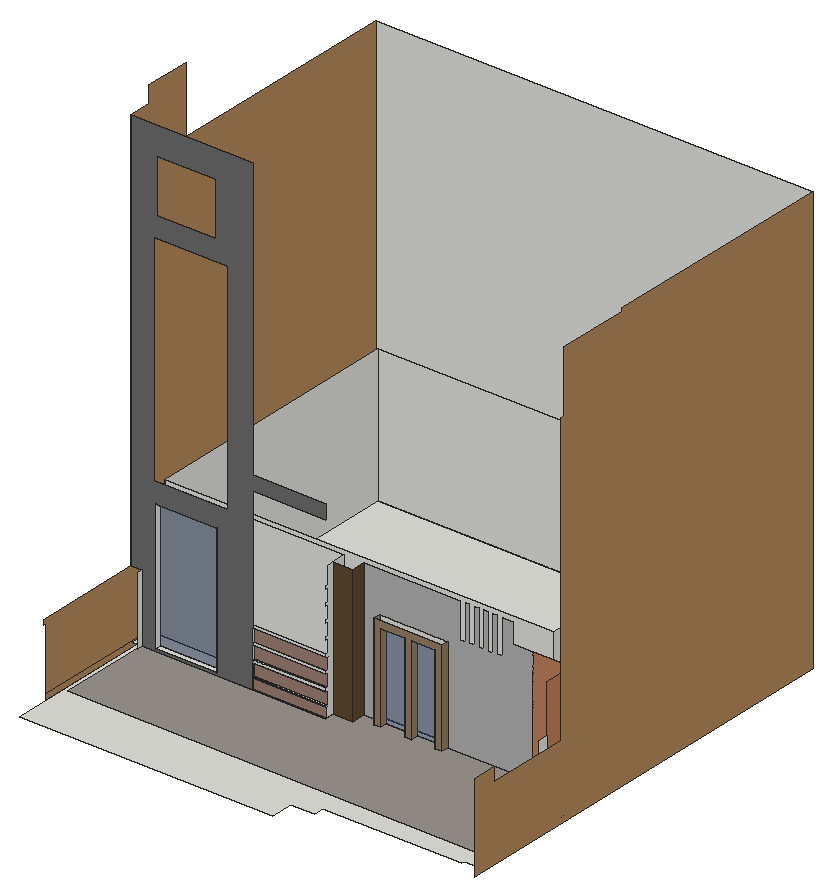
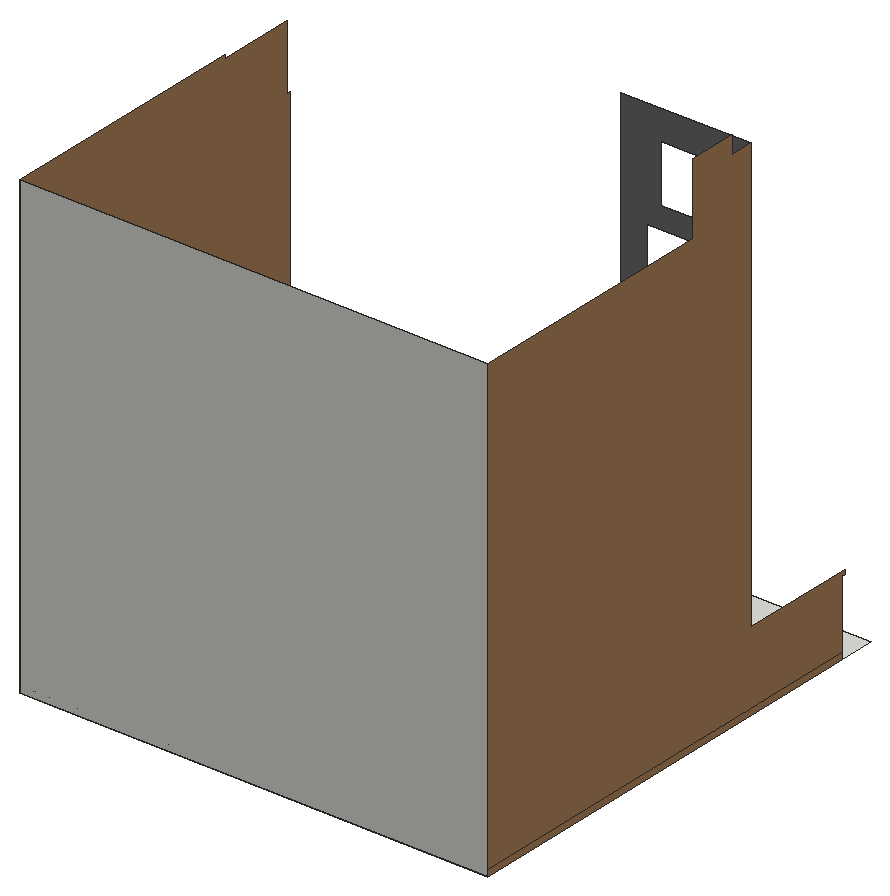
# SketchUp Ruby script. Lengths in inches.
U = 1.inch
M = Sketchup.active_model
def pt(a) = Geom::Point3d.new(a.map { |v| v * U })
def face(e, loops, mat)
  f = e.add_face(loops[0].map { |a| pt(a) })
  loops[1..].each { |l| e.add_face(l.map { |a| pt(a) }).erase! }
  f.material = f.back_material = mat if mat
  f
end
# faces: each face lists its corners as indices into pts; further lists are holes
def faces(e, pts, list, mat = nil) = list.each { |f| face(e, (f[0].is_a?(Array) ? f : [f]).map { |l| l.map { |i| pts[i] } }, mat) }
# xy, xz, yz: faces in a plane at the given z, y or x. An outline is a flat list of corners, or four numbers for a rectangle; further outlines are holes
def ring(l) = l.size == 4 ? [[l[0], l[1]], [l[2], l[1]], [l[2], l[3]], [l[0], l[3]]] : l.each_slice(2).to_a
def flat(e, list, mat, &to3) = list.each { |f| face(e, (f[0].is_a?(Array) ? f : [f]).map { |l| ring(l).map { |u, v| to3.(u, v) } }, mat) }
def xy(e, z, list, mat = nil) = flat(e, list, mat) { |x, y| [x, y, z] }
def xz(e, y, list, mat = nil) = flat(e, list, mat) { |x, z| [x, y, z] }
def yz(e, x, list, mat = nil) = flat(e, list, mat) { |y, z| [x, y, z] }
def lines(e, pts, list) = list.each { |a, b| e.add_line(pt(pts[a]), pt(pts[b])) }
# prism: a flat outline (further loops are holes) pulled along v
def prism(e, loops, v, mat = nil)
  f = face(e, loops, mat); d = Geom::Vector3d.new(v.map { |x| x * U })
  f.pushpull(f.normal.samedirection?(d) ? d.length : -d.length)
end
def box(e, o, s, mat = nil) = prism(e, [[o, [o[0] + s[0], o[1], o[2]], [o[0] + s[0], o[1] + s[1], o[2]], [o[0], o[1] + s[1], o[2]]]], [0, 0, s[2]], mat)
def at(x, y, z, deg = 0) = Geom::Transformation.translation(pt([x, y, z])) * Geom::Transformation.rotation(ORIGIN, Z_AXIS, deg.degrees)
def axes(o, x, y, z) = Geom::Transformation.new([*x, 0, *y, 0, *z, 0, *pt(o).to_a, 1])
def part(name) = M.definitions.add(name)
# library, detail: a bought-in or finely detailed component or shape, given as its bounding box
def library(name, o, s) = part(name).tap { |d| box(d.entities, o, s) }
def detail(e, o, s) = box(e.add_group.entities, o, s)
def put(e, d, t, mat = nil) = e.add_instance(d, t).tap { |i| i.material = mat if mat }
def group(e, t, mat = nil) = e.add_group.tap { |g| g.transformation = t; g.material = mat if mat }.entities
root = M.entities
M.materials.add("Niraj_Hair_Dark").color = [109, 109, 109]
M.materials.add("Niraj_Hair_Gray").color = [178, 178, 178]
M.materials.add("Niraj_Shoe_Sole").color = [96, 73, 48]
M.materials.add("Niraj_Shoe_Stitching").color = [181, 137, 92]
M.materials.add("Niraj_Skin").color = [158, 128, 115]
M.materials.add("[0035_Tan]").color = [150, 128, 100]
M.materials.add("[Granite Tile]").color = [155, 148, 143]
M.materials.add("[Translucent Glass Blue]").color = [40, 60, 96]
M.materials["[Translucent Glass Blue]"].alpha = 0.5
M.materials.add("[Translucent Glass Blue]1").color = [46, 68, 109]
M.materials["[Translucent Glass Blue]1"].alpha = 0.5
M.materials.add("[Wood Veneer 02]").color = [190, 128, 91]
xy(root,-4.9375,[[0,0,0,391.875,372,391.875,372,115,384,115,384,31.875,365.58,31.875,365.58,28.875,243.65,28.875,243.65,19.875,222.65,19.875,222.65,0],[372,115,384,118],[372,118,384,142],[372,142,372,143.6875,373.25,143.6875,373.25,391.875,384,391.875,384,142],[372,143.6875,373.25,391.875]])
xy(root,0,[[0,122.375,9,142],[9,122.375,106.63,122.375,106.63,123.4375,171.63,123.4375,171.63,142,9,142],[106.63,122.375,171.63,123.1875],[106.63,123.1875,171.63,123.4375],[202.6,136,203.04,142],
  [203.04,136,208.6,142],[229.96,136,231.09,142],[231.09,136,235.96,142],[256.6,136,262.6,142],[262.6,142,337.38,143.6875],
  [337.38,142,360,143.6875],[360,142,360.25,143.6875],[360.25,142,372,143.6875],[262.6,143.6875,337.38,148],[9,148,262.6,382.875],
  [262.6,148,337.38,382.875],[337.38,148,351,382.875]])
xy(root,0,[[9,40.875,375,40.875,375,106,372,106,372,142,262.6,142,262.6,136,256.6,136,256.6,142,235.96,142,235.96,136,229.96,136,229.96,142,208.6,142,208.6,136,202.6,136,202.6,142,189.04,142,189.04,130,171.63,130,171.63,122.375,9,122.375]],"[Granite Tile]")
xy(root,2,[[21.24,122.375,75.18,127.1875]])
xy(root,9.02,[[106.63,122.375,171.63,123.1875]])
xy(root,10.2,[[106.63,122.375,171.63,123.625],[106.63,123.625,171.63,123.75]])
xy(root,21.27,[[106.63,122.375,171.63,123.625],[106.63,123.625,171.63,123.75]])
xy(root,23.7,[[106.63,122.375,171.63,124.125],[106.63,124.125,171.63,124.1875]])
xy(root,34.77,[[106.63,122.375,171.63,124.125],[106.63,124.125,171.63,124.1875]])
xy(root,37.2,[[106.63,122.375,171.63,123.5625]])
xy(root,48.27,[[106.63,122.375,171.63,123.5625]])
xz(root,122.375,[[106.63,-2.05,171.63,0],[106.63,9.02,171.63,10.2],[106.63,21.27,171.63,23.7],[106.63,34.77,171.63,37.2],[106.63,48.27,171.63,50.7]])
xz(root,122.375,[[[9,0,106.63,0,106.63,156.27,171.63,156.27,171.63,169.15,106.63,169.15,106.63,415.46,0,415.46,0,60,9,60],[20.16,134.02,85.33,326.3125],[21.24,2,75.18,116.62],[22.76,343.6,74.01,391.1]]],"Niraj_Hair_Dark")
xz(root,123.1875,[[106.63,0,171.63,9.02]],"Niraj_Skin")
xz(root,123.5625,[[106.63,37.2,171.63,48.27]],"Niraj_Skin")
xz(root,123.75,[[106.63,10.2,171.63,21.27]],"Niraj_Skin")
xz(root,124.1875,[[106.63,23.7,171.63,34.77]],"Niraj_Skin")
xz(root,127.1875,[[21.24,2,75.18,116.62]],"[Translucent Glass Blue]")
xz(root,130,[[171.63,0,189.04,120]],"Niraj_Shoe_Sole")
xz(root,136,[[202.6,0,208.6,0,208.6,78,229.96,78,229.96,0,235.96,0,235.96,78,256.6,78,256.6,0,262.6,0,262.6,84,202.6,84]],"[0035_Tan]")
xz(root,142,[[9,0,171.63,120],[202.6,0,202.6,84,262.6,84,262.6,0,256.6,0,256.6,78,235.96,78,235.96,0,229.96,0,229.96,78,208.6,78,208.6,0]])
xz(root,142,[[189.04,0,202.6,0,202.6,84,262.6,84,262.6,0,337.38,0,337.38,102.25,320.38,102.25,320.38,120,311.1,120,311.1,89.375,306.22,89.375,306.22,120,302.91,120,302.91,89.375,298.04,89.375,298.04,120,294.72,120,294.72,89.375,289.85,89.375,289.85,120,286.54,120,286.54,89.375,281.66,89.375,281.66,120,278.35,120,278.35,89.375,273.47,89.375,273.47,120,189.04,120]],"Niraj_Hair_Gray")
xz(root,142,[[208.6,0,229.96,78],[235.96,0,256.6,78]],"[Translucent Glass Blue]1")
xz(root,142,[[337.38,0,372,102.25]],"[Wood Veneer 02]")
xz(root,143.6875,[[372,-4.9375,373.25,0]])
xz(root,148,[[9,0,351,120]])
xz(root,382.875,[[9,-4.9375,262.6,0],[9,0,351,120]])
xz(root,391.875,[[0,-4.9375,384,371.75]])
yz(root,0,[[28.875,-4.9375,391.875,0],[28.875,0,28.875,56.2,25.875,56.2,25.875,60,122.375,60,122.375,415.46,142,415.46,142,430.21,182.0625,430.21,182.0625,371.75,391.875,371.75,391.875,0]],"Niraj_Shoe_Stitching")
yz(root,9,[[117.875,0,122.375,60],[148,0,382.875,120]])
yz(root,21.24,[[122.375,2,127.1875,116.62]])
yz(root,75.18,[[122.375,2,127.1875,116.62]])
yz(root,106.63,[[122.375,0,123.1875,9.02],[123.1875,0,123.4375,9.02],[122.375,10.2,123.625,21.27],[123.625,10.2,123.75,21.27],[122.375,23.7,124.125,34.77],
  [124.125,23.7,124.1875,34.77],[122.375,37.2,123.5625,48.27],[123.5625,37.2,124.25,48.27]])
yz(root,171.63,[[123.1875,0,130,0,130,120,123.6875,120,123.6875,118.2,124.1875,118.2,124.1875,104.7,122.375,104.7,122.375,102.27,123.5,102.27,123.5,91.2,122.375,91.2,122.375,88.77,123.5625,88.77,123.5625,77.7,122.375,77.7,122.375,75.27,123.875,75.27,123.875,64.2,122.375,64.2,122.375,61.77,124.5,61.77,124.5,50.7,122.375,50.7,122.375,48.27,123.5625,48.27,123.5625,37.2,122.375,37.2,122.375,34.77,124.1875,34.77,124.1875,23.7,122.375,23.7,122.375,21.27,123.75,21.27,123.75,10.2,122.375,10.2,122.375,9.02,123.1875,9.02],[130,0,142,120]])
yz(root,189.04,[[130,0,142,120]],"Niraj_Shoe_Sole")
yz(root,202.6,[[136,0,142,84]],"[0035_Tan]")
yz(root,208.6,[[136,0,142,78]],"[0035_Tan]")
yz(root,229.96,[[136,0,142,78]],"[0035_Tan]")
yz(root,235.96,[[136,0,142,78]],"[0035_Tan]")
yz(root,256.6,[[136,0,142,78]],"[0035_Tan]")
yz(root,262.6,[[136,0,142,84]],"[0035_Tan]")
yz(root,351,[[148,0,382.875,120]])
yz(root,372,[[115,-4.9375,118,0],[118,-4.9375,142,0],[142,-4.9375,143.6875,0],[106,0,115,60],[142,0,143.6875,0.625]])
yz(root,372,[[115,0,142,102.25]],"[Wood Veneer 02]")
yz(root,384,[[19.875,-4.9375,391.875,-4.9375,391.875,371.75,182.0625,371.75,182.0625,369.0625,118,369.0625,118,314.9,115,314.9,115,60,40.875,60,40.875,72,19.875,72]],"Niraj_Shoe_Stitching")
p = [[106.63,124.25,48.27],[171.63,124.25,48.27],[106.63,123.4375,9.02],[171.63,123.4375,9.02],[372,118,0],[384,118,0],
  [360,143.6875,0],[360,391.875,0],[337.38,382.875,0],[337.38,391.875,0],[262.6,382.875,0],[262.6,391.875,0],
  [372,143.6875,0.625],[372,391.875,0.625],[373.25,143.6875,0],[373.25,391.875,0],[9,148,0],[9,148,-4.9375],
  [9,117.875,0],[9,117.875,-4.9375],[9,142,0],[9,142,-4.9375],[262.6,382.875,-4.9375],[262.6,391.875,-4.9375],
  [202.6,142,0],[202.6,142,-4.9375],[372,115,0],[384,115,0]]
lines(root,p,[[0,1],[2,3],[4,5],[6,7],[8,9],[10,11],[12,13],[14,15],[16,17],[18,19],[20,21],[22,23],
  [24,25],[26,27]])
